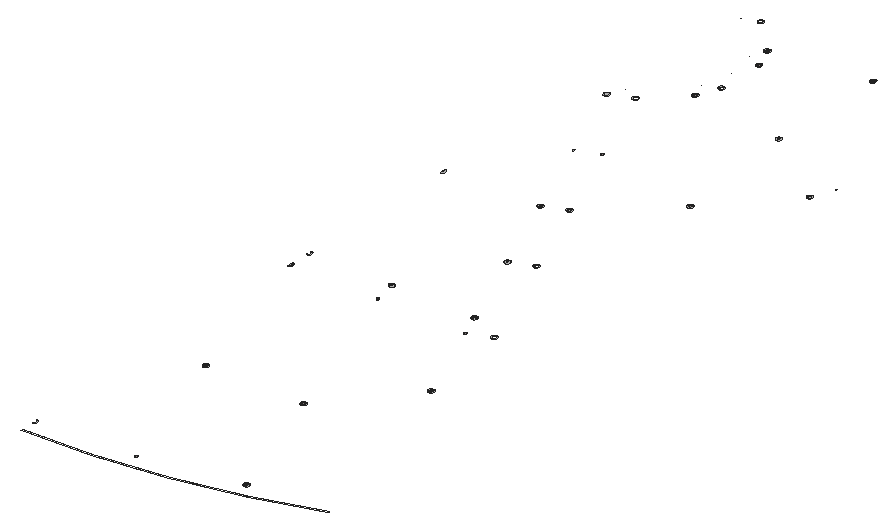
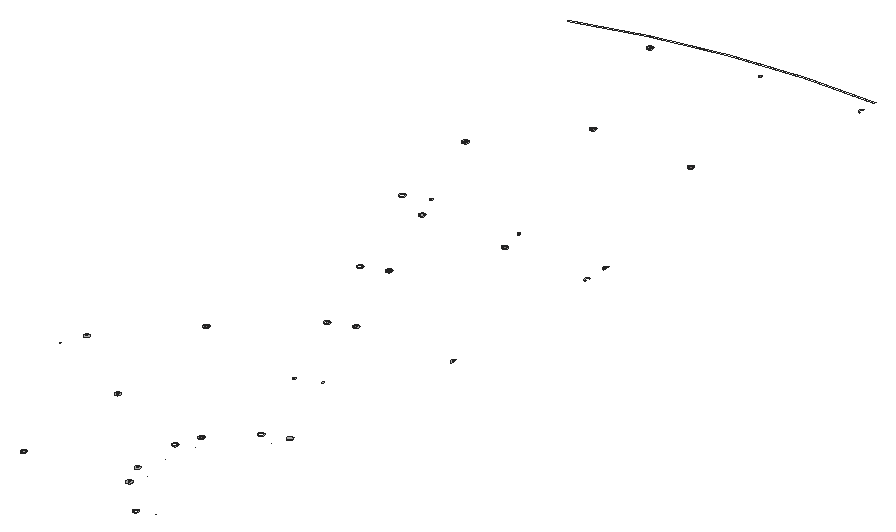
# SketchUp Ruby script. Lengths in inches.
U = 1.inch
M = Sketchup.active_model
def pt(a) = Geom::Point3d.new(a.map { |v| v * U })
def face(e, loops, mat)
  f = e.add_face(loops[0].map { |a| pt(a) })
  loops[1..].each { |l| e.add_face(l.map { |a| pt(a) }).erase! }
  f.material = f.back_material = mat if mat
  f
end
# faces: each face lists its corners as indices into pts; further lists are holes
def faces(e, pts, list, mat = nil) = list.each { |f| face(e, (f[0].is_a?(Array) ? f : [f]).map { |l| l.map { |i| pts[i] } }, mat) }
# xy, xz, yz: faces in a plane at the given z, y or x. An outline is a flat list of corners, or four numbers for a rectangle; further outlines are holes
def ring(l) = l.size == 4 ? [[l[0], l[1]], [l[2], l[1]], [l[2], l[3]], [l[0], l[3]]] : l.each_slice(2).to_a
def flat(e, list, mat, &to3) = list.each { |f| face(e, (f[0].is_a?(Array) ? f : [f]).map { |l| ring(l).map { |u, v| to3.(u, v) } }, mat) }
def xy(e, z, list, mat = nil) = flat(e, list, mat) { |x, y| [x, y, z] }
def xz(e, y, list, mat = nil) = flat(e, list, mat) { |x, z| [x, y, z] }
def yz(e, x, list, mat = nil) = flat(e, list, mat) { |y, z| [x, y, z] }
def lines(e, pts, list) = list.each { |a, b| e.add_line(pt(pts[a]), pt(pts[b])) }
# prism: a flat outline (further loops are holes) pulled along v
def prism(e, loops, v, mat = nil)
  f = face(e, loops, mat); d = Geom::Vector3d.new(v.map { |x| x * U })
  f.pushpull(f.normal.samedirection?(d) ? d.length : -d.length)
end
def box(e, o, s, mat = nil) = prism(e, [[o, [o[0] + s[0], o[1], o[2]], [o[0] + s[0], o[1] + s[1], o[2]], [o[0], o[1] + s[1], o[2]]]], [0, 0, s[2]], mat)
def at(x, y, z, deg = 0) = Geom::Transformation.translation(pt([x, y, z])) * Geom::Transformation.rotation(ORIGIN, Z_AXIS, deg.degrees)
def axes(o, x, y, z) = Geom::Transformation.new([*x, 0, *y, 0, *z, 0, *pt(o).to_a, 1])
def part(name) = M.definitions.add(name)
# library, detail: a bought-in or finely detailed component or shape, given as its bounding box
def library(name, o, s) = part(name).tap { |d| box(d.entities, o, s) }
def detail(e, o, s) = box(e.add_group.entities, o, s)
def put(e, d, t, mat = nil) = e.add_instance(d, t).tap { |i| i.material = mat if mat }
def group(e, t, mat = nil) = e.add_group.tap { |g| g.transformation = t; g.material = mat if mat }.entities
root = M.entities
M.materials.add("[Asphalt_Stamped_Brick]").color = [149, 133, 134]
M.materials.add("[Metal_Steel_Textured_White]").color = [191, 191, 191]
xy(root,3.625,[[153.108,137.349,153.103,137.35,153.098,137.352,153.094,137.355,153.09,137.359,153.088,137.364,153.088,137.374,153.09,137.379,153.098,137.387,153.103,137.389,153.113,137.389,153.118,137.387,153.122,137.383,153.125,137.379,153.127,137.374,153.128,137.369,153.127,137.364,153.125,137.359,153.122,137.355,153.118,137.352,153.113,137.35],[156.34,137.968,156.336,137.97,156.331,137.974,156.328,137.978,156.326,137.983,156.326,137.993,156.328,137.998,156.331,138.002,156.336,138.005,156.34,138.007,156.345,138.008,156.351,138.007,156.355,138.005,156.36,138.002,156.363,137.998,156.365,137.993,156.365,137.983,156.363,137.978,156.36,137.974,156.355,137.97,156.351,137.968],[151.473,142.332,151.468,142.333,151.463,142.335,151.459,142.338,151.456,142.342,151.454,142.347,151.453,142.352,151.454,142.357,151.456,142.362,151.459,142.366,151.463,142.369,151.468,142.371,151.473,142.372,151.478,142.371,151.483,142.369,151.487,142.366,151.491,142.362,151.493,142.357,151.493,142.347,151.491,142.342,151.487,142.338,151.483,142.335,151.478,142.333],[154.784,142.332,154.779,142.333,154.774,142.335,154.77,142.338,154.767,142.342,154.765,142.347,154.764,142.352,154.765,142.357,154.767,142.362,154.77,142.366,154.774,142.369,154.779,142.371,154.784,142.372,154.789,142.371,154.794,142.369,154.798,142.366,154.801,142.362,154.803,142.357,154.804,142.352,154.803,142.347,154.801,142.342,154.798,142.338,154.794,142.335,154.789,142.333],[156.99,144.988,156.985,144.99,156.981,144.993,156.978,144.998,156.976,145.002,156.975,145.008,156.976,145.013,156.978,145.018,156.981,145.022,156.985,145.025,156.99,145.027,156.995,145.028,157,145.027,157.005,145.025,157.009,145.022,157.012,145.018,157.014,145.013,157.015,145.008,157.014,145.002,157.012,144.998,157.009,144.993,157.005,144.99,157,144.988],
  [152.78,147.988,152.775,147.99,152.771,147.993,152.768,147.998,152.766,148.002,152.765,148.008,152.766,148.013,152.768,148.018,152.771,148.022,152.775,148.025,152.78,148.027,152.79,148.027,152.795,148.025,152.799,148.022,152.802,148.018,152.804,148.013,152.805,148.008,152.804,148.002,152.802,147.998,152.799,147.993,152.795,147.99,152.79,147.988],[155.747,147.988,155.742,147.99,155.738,147.993,155.735,147.998,155.733,148.002,155.732,148.008,155.733,148.013,155.735,148.018,155.738,148.022,155.742,148.025,155.747,148.027,155.757,148.027,155.762,148.025,155.766,148.022,155.769,148.018,155.771,148.013,155.772,148.008,155.771,148.002,155.769,147.998,155.766,147.993,155.762,147.99,155.757,147.988],[152.62,148.786,152.615,148.787,152.61,148.789,152.606,148.792,152.602,148.796,152.6,148.801,152.6,148.811,152.602,148.816,152.606,148.82,152.61,148.823,152.615,148.825,152.62,148.826,152.625,148.825,152.63,148.823,152.634,148.82,152.637,148.816,152.639,148.811,152.64,148.806,152.639,148.801,152.637,148.796,152.634,148.792,152.63,148.789,152.625,148.787],[153.011,154.594,153.006,154.596,153.002,154.599,152.999,154.604,152.997,154.608,152.996,154.614,152.997,154.619,152.999,154.624,153.002,154.628,153.006,154.631,153.011,154.633,153.021,154.633,153.026,154.631,153.03,154.628,153.033,154.624,153.035,154.619,153.036,154.614,153.035,154.608,153.033,154.604,153.03,154.599,153.026,154.596,153.021,154.594],[156.122,157.053,156.117,157.054,156.112,157.056,156.108,157.059,156.105,157.063,156.103,157.068,156.102,157.073,156.103,157.078,156.105,157.083,156.108,157.087,156.112,157.09,156.117,157.092,156.122,157.093,156.128,157.092,156.132,157.09,156.136,157.087,156.14,157.083,156.142,157.078,156.142,157.068,156.14,157.063,156.136,157.059,156.132,157.056,156.128,157.054],
  [152.551,157.803,152.546,157.804,152.541,157.806,152.537,157.809,152.533,157.813,152.531,157.818,152.531,157.828,152.533,157.833,152.537,157.837,152.541,157.84,152.546,157.842,152.551,157.843,152.556,157.842,152.561,157.84,152.565,157.837,152.568,157.833,152.57,157.828,152.571,157.823,152.57,157.818,152.568,157.813,152.565,157.809,152.561,157.806,152.556,157.804],[158.582,160.159,158.577,160.16,158.572,160.162,158.568,160.165,158.564,160.169,158.5625,160.174,158.562,160.179,158.5625,160.185,158.564,160.189,158.568,160.194,158.572,160.197,158.577,160.199,158.587,160.199,158.592,160.197,158.596,160.194,158.599,160.189,158.601,160.185,158.602,160.179,158.601,160.174,158.599,160.169,158.596,160.165,158.592,160.162,158.587,160.16],[155.678,161.362,155.673,161.363,155.668,161.365,155.664,161.368,155.661,161.372,155.659,161.377,155.658,161.382,155.659,161.387,155.661,161.392,155.664,161.396,155.668,161.399,155.673,161.401,155.678,161.402,155.683,161.401,155.688,161.399,155.692,161.396,155.695,161.392,155.697,161.387,155.698,161.382,155.697,161.377,155.695,161.372,155.692,161.368,155.688,161.365,155.683,161.363],[152.469,161.827,152.463,161.828,152.459,161.83,152.455,161.833,152.451,161.837,152.449,161.842,152.449,161.852,152.451,161.857,152.459,161.865,152.463,161.867,152.474,161.867,152.479,161.865,152.483,161.861,152.486,161.857,152.488,161.852,152.489,161.847,152.488,161.842,152.486,161.837,152.483,161.833,152.479,161.83,152.474,161.828],[152.774,164.15,152.769,164.151,152.764,164.153,152.76,164.156,152.757,164.16,152.755,164.165,152.754,164.17,152.755,164.175,152.757,164.18,152.76,164.184,152.764,164.187,152.769,164.189,152.774,164.19,152.779,164.189,152.784,164.187,152.788,164.184,152.791,164.18,152.793,164.175,152.794,164.17,152.793,164.165,152.791,164.16,152.788,164.156,152.784,164.153,152.779,164.151]],"[Asphalt_Stamped_Brick]")
xy(root,3.625,[[149.818,137.073,149.818,137.074,149.841,137.077,149.862,137.086,149.88,137.1,149.894,137.118,149.903,137.139,149.906,137.162,149.903,137.185,149.894,137.206,149.88,137.224,149.862,137.238,149.841,137.247,149.818,137.25,149.818,137.251,149.841,137.248,149.862,137.239,149.881,137.225,149.895,137.207,149.904,137.185,149.907,137.162,149.904,137.139,149.895,137.118,149.881,137.099,149.862,137.085,149.841,137.076],[[153.108,137.333,153.098,137.334,153.089,137.338,153.082,137.343,153.076,137.351,153.072,137.36,153.071,137.369,153.072,137.379,153.076,137.388,153.082,137.395,153.089,137.401,153.098,137.405,153.108,137.406,153.117,137.405,153.126,137.401,153.134,137.395,153.139,137.388,153.143,137.379,153.144,137.369,153.143,137.36,153.139,137.351,153.134,137.343,153.126,137.338,153.117,137.334],[153.108,137.349,153.113,137.35,153.118,137.352,153.122,137.355,153.125,137.359,153.127,137.364,153.128,137.369,153.127,137.374,153.125,137.379,153.122,137.383,153.118,137.387,153.113,137.389,153.103,137.389,153.098,137.387,153.09,137.379,153.088,137.374,153.088,137.364,153.09,137.359,153.094,137.355,153.098,137.352,153.103,137.35]],[[156.345,137.899,156.322,137.902,156.301,137.911,156.283,137.925,156.269,137.943,156.26,137.965,156.257,137.988,156.26,138.011,156.269,138.032,156.283,138.051,156.301,138.065,156.322,138.074,156.345,138.077,156.368,138.074,156.39,138.065,156.408,138.051,156.422,138.032,156.431,138.011,156.434,137.988,156.431,137.965,156.422,137.943,156.408,137.925,156.39,137.911,156.368,137.902],[156.345,137.9,156.368,137.903,156.389,137.912,156.408,137.926,156.422,137.944,156.43,137.965,156.433,137.988,156.43,138.011,156.422,138.032,156.408,138.05,156.389,138.064,156.368,138.073,156.345,138.076,156.323,138.073,156.302,138.064,156.283,138.05,156.269,138.032,156.261,138.011,156.258,137.988,156.261,137.965,156.269,137.944,156.283,137.926,156.302,137.912,156.323,137.903]],[[156.345,137.9,156.323,137.903,156.302,137.912,156.283,137.926,156.269,137.944,156.261,137.965,156.258,137.988,156.261,138.011,156.269,138.032,156.283,138.05,156.302,138.064,156.323,138.073,156.345,138.076,156.368,138.073,156.389,138.064,156.408,138.05,156.422,138.032,156.43,138.011,156.433,137.988,156.43,137.965,156.422,137.944,156.408,137.926,156.389,137.912,156.368,137.903],[156.345,137.951,156.355,137.952,156.364,137.956,156.371,137.962,156.377,137.969,156.381,137.978,156.382,137.988,156.381,137.997,156.377,138.006,156.371,138.014,156.364,138.019,156.355,138.023,156.345,138.024,156.336,138.023,156.327,138.019,156.32,138.014,156.314,138.006,156.31,137.997,156.309,137.988,156.31,137.978,156.314,137.969,156.32,137.962,156.327,137.956,156.336,137.952]],[[156.345,137.951,156.336,137.952,156.327,137.956,156.32,137.962,156.314,137.969,156.31,137.978,156.309,137.988,156.31,137.997,156.314,138.006,156.32,138.014,156.327,138.019,156.336,138.023,156.345,138.024,156.355,138.023,156.364,138.019,156.371,138.014,156.377,138.006,156.381,137.997,156.382,137.988,156.381,137.978,156.377,137.969,156.371,137.962,156.364,137.956,156.355,137.952],[156.34,137.968,156.351,137.968,156.355,137.97,156.36,137.974,156.363,137.978,156.365,137.983,156.365,137.993,156.363,137.998,156.36,138.002,156.355,138.005,156.351,138.007,156.345,138.008,156.34,138.007,156.336,138.005,156.331,138.002,156.328,137.998,156.326,137.993,156.326,137.983,156.328,137.978,156.331,137.974,156.336,137.97]],
  [[151.473,142.263,151.45,142.266,151.429,142.275,151.41,142.289,151.396,142.307,151.387,142.329,151.384,142.352,151.387,142.375,151.396,142.396,151.41,142.415,151.429,142.429,151.45,142.438,151.473,142.441,151.496,142.438,151.518,142.429,151.536,142.415,151.55,142.396,151.559,142.375,151.562,142.352,151.559,142.329,151.55,142.307,151.536,142.289,151.518,142.275,151.496,142.266],[151.473,142.264,151.496,142.267,151.517,142.276,151.535,142.29,151.549,142.308,151.558,142.329,151.561,142.352,151.558,142.375,151.549,142.396,151.535,142.414,151.517,142.428,151.496,142.437,151.473,142.44,151.451,142.437,151.429,142.428,151.411,142.414,151.397,142.396,151.388,142.375,151.385,142.352,151.388,142.329,151.397,142.308,151.411,142.29,151.429,142.276,151.451,142.267]],[[154.784,142.263,154.761,142.266,154.74,142.275,154.721,142.289,154.707,142.307,154.698,142.329,154.695,142.352,154.698,142.375,154.707,142.396,154.721,142.415,154.74,142.429,154.761,142.438,154.784,142.441,154.807,142.438,154.828,142.429,154.847,142.415,154.861,142.396,154.87,142.375,154.873,142.352,154.87,142.329,154.861,142.307,154.847,142.289,154.828,142.275,154.807,142.266],[154.784,142.264,154.807,142.267,154.828,142.276,154.846,142.29,154.86,142.308,154.869,142.329,154.872,142.352,154.869,142.375,154.86,142.396,154.846,142.414,154.828,142.428,154.807,142.437,154.784,142.44,154.761,142.437,154.74,142.428,154.722,142.414,154.708,142.396,154.699,142.375,154.696,142.352,154.699,142.329,154.708,142.308,154.722,142.29,154.74,142.276,154.761,142.267]],[[151.473,142.264,151.451,142.267,151.429,142.276,151.411,142.29,151.397,142.308,151.388,142.329,151.385,142.352,151.388,142.375,151.397,142.396,151.411,142.414,151.429,142.428,151.451,142.437,151.473,142.44,151.496,142.437,151.517,142.428,151.535,142.414,151.549,142.396,151.558,142.375,151.561,142.352,151.558,142.329,151.549,142.308,151.535,142.29,151.517,142.276,151.496,142.267],[151.473,142.315,151.483,142.317,151.492,142.32,151.499,142.326,151.505,142.334,151.509,142.342,151.51,142.352,151.509,142.361,151.505,142.37,151.499,142.378,151.492,142.384,151.483,142.387,151.473,142.389,151.464,142.387,151.455,142.384,151.447,142.378,151.442,142.37,151.438,142.361,151.437,142.352,151.438,142.342,151.442,142.334,151.447,142.326,151.455,142.32,151.464,142.317]],[[151.473,142.315,151.464,142.317,151.455,142.32,151.447,142.326,151.442,142.334,151.438,142.342,151.437,142.352,151.438,142.361,151.442,142.37,151.447,142.378,151.455,142.384,151.464,142.387,151.473,142.389,151.483,142.387,151.492,142.384,151.499,142.378,151.505,142.37,151.509,142.361,151.51,142.352,151.509,142.342,151.505,142.334,151.499,142.326,151.492,142.32,151.483,142.317],[151.473,142.332,151.478,142.333,151.483,142.335,151.487,142.338,151.491,142.342,151.493,142.347,151.493,142.357,151.491,142.362,151.487,142.366,151.483,142.369,151.478,142.371,151.473,142.372,151.468,142.371,151.463,142.369,151.459,142.366,151.456,142.362,151.454,142.357,151.453,142.352,151.454,142.347,151.456,142.342,151.459,142.338,151.463,142.335,151.468,142.333]],[[154.784,142.315,154.775,142.317,154.766,142.32,154.758,142.326,154.752,142.334,154.749,142.342,154.747,142.352,154.749,142.361,154.752,142.37,154.758,142.378,154.766,142.384,154.775,142.387,154.784,142.389,154.794,142.387,154.802,142.384,154.81,142.378,154.816,142.37,154.819,142.361,154.821,142.352,154.819,142.342,154.816,142.334,154.81,142.326,154.802,142.32,154.794,142.317],[154.784,142.332,154.789,142.333,154.794,142.335,154.798,142.338,154.801,142.342,154.803,142.347,154.804,142.352,154.803,142.357,154.801,142.362,154.798,142.366,154.794,142.369,154.789,142.371,154.784,142.372,154.779,142.371,154.774,142.369,154.77,142.366,154.767,142.362,154.765,142.357,154.764,142.352,154.765,142.347,154.767,142.342,154.77,142.338,154.774,142.335,154.779,142.333]],
  [[156.995,144.919,156.972,144.922,156.95,144.931,156.932,144.945,156.918,144.963,156.909,144.985,156.906,145.008,156.909,145.031,156.918,145.052,156.932,145.07,156.95,145.085,156.972,145.093,156.995,145.096,157.018,145.093,157.039,145.085,157.058,145.07,157.072,145.052,157.081,145.031,157.084,145.008,157.081,144.985,157.072,144.963,157.058,144.945,157.039,144.931,157.018,144.922],[156.995,144.92,157.018,144.923,157.039,144.931,157.057,144.945,157.071,144.964,157.08,144.985,157.083,145.008,157.08,145.03,157.071,145.052,157.057,145.07,157.039,145.084,157.018,145.092,156.995,145.095,156.972,145.092,156.951,145.084,156.933,145.07,156.919,145.052,156.91,145.03,156.907,145.008,156.91,144.985,156.919,144.964,156.933,144.945,156.951,144.931,156.972,144.923]],[[156.995,144.971,156.985,144.972,156.977,144.976,156.969,144.982,156.963,144.989,156.959,144.998,156.958,145.008,156.959,145.017,156.963,145.026,156.969,145.033,156.977,145.039,156.985,145.043,156.995,145.044,157.004,145.043,157.013,145.039,157.021,145.033,157.027,145.026,157.03,145.017,157.031,145.008,157.03,144.998,157.027,144.989,157.021,144.982,157.013,144.976,157.004,144.972],[156.99,144.988,157,144.988,157.005,144.99,157.009,144.993,157.012,144.998,157.014,145.002,157.015,145.008,157.014,145.013,157.012,145.018,157.009,145.022,157.005,145.025,157,145.027,156.995,145.028,156.99,145.027,156.985,145.025,156.981,145.022,156.978,145.018,156.976,145.013,156.975,145.008,156.976,145.002,156.978,144.998,156.981,144.993,156.985,144.99]],[149.818,147.919,149.818,147.92,149.841,147.923,149.862,147.931,149.88,147.945,149.894,147.964,149.903,147.985,149.906,148.008,149.903,148.03,149.894,148.051,149.88,148.07,149.862,148.084,149.841,148.092,149.818,148.095,149.818,148.096,149.841,148.093,149.862,148.085,149.881,148.07,149.895,148.052,149.904,148.031,149.907,148.008,149.904,147.985,149.895,147.963,149.881,147.945,149.862,147.931,149.841,147.922],[[152.785,147.971,152.776,147.972,152.767,147.976,152.759,147.982,152.753,147.989,152.75,147.998,152.748,148.008,152.75,148.017,152.753,148.026,152.759,148.033,152.767,148.039,152.776,148.043,152.785,148.044,152.795,148.043,152.803,148.039,152.811,148.033,152.817,148.026,152.82,148.017,152.822,148.008,152.82,147.998,152.817,147.989,152.811,147.982,152.803,147.976,152.795,147.972],[152.78,147.988,152.79,147.988,152.795,147.99,152.799,147.993,152.802,147.998,152.804,148.002,152.805,148.008,152.804,148.013,152.802,148.018,152.799,148.022,152.795,148.025,152.79,148.027,152.78,148.027,152.775,148.025,152.771,148.022,152.768,148.018,152.766,148.013,152.765,148.008,152.766,148.002,152.768,147.998,152.771,147.993,152.775,147.99]],[[155.752,147.971,155.743,147.972,155.734,147.976,155.726,147.982,155.721,147.989,155.717,147.998,155.716,148.008,155.717,148.017,155.721,148.026,155.726,148.033,155.734,148.039,155.743,148.043,155.752,148.044,155.762,148.043,155.771,148.039,155.778,148.033,155.784,148.026,155.788,148.017,155.789,148.008,155.788,147.998,155.784,147.989,155.778,147.982,155.771,147.976,155.762,147.972],[155.747,147.988,155.757,147.988,155.762,147.99,155.766,147.993,155.769,147.998,155.771,148.002,155.772,148.008,155.771,148.013,155.769,148.018,155.766,148.022,155.762,148.025,155.757,148.027,155.747,148.027,155.742,148.025,155.738,148.022,155.735,148.018,155.733,148.013,155.732,148.008,155.733,148.002,155.735,147.998,155.738,147.993,155.742,147.99]],
  [149.818,147.988,149.818,148.027,149.823,148.027,149.828,148.025,149.832,148.022,149.835,148.018,149.837,148.013,149.838,148.008,149.837,148.002,149.835,147.998,149.832,147.993,149.828,147.99,149.823,147.988],[[156.49,148.224,156.467,148.227,156.445,148.236,156.427,148.25,156.413,148.269,156.404,148.29,156.401,148.313,156.404,148.336,156.413,148.358,156.427,148.376,156.445,148.39,156.467,148.399,156.49,148.402,156.513,148.399,156.534,148.39,156.553,148.376,156.567,148.358,156.576,148.336,156.579,148.313,156.576,148.29,156.567,148.269,156.553,148.25,156.534,148.236,156.513,148.227],[156.49,148.225,156.513,148.228,156.534,148.237,156.552,148.251,156.566,148.269,156.575,148.29,156.578,148.313,156.575,148.336,156.566,148.357,156.552,148.375,156.534,148.389,156.513,148.398,156.49,148.401,156.467,148.398,156.446,148.389,156.428,148.375,156.414,148.357,156.405,148.336,156.402,148.313,156.405,148.29,156.414,148.269,156.428,148.251,156.446,148.237,156.467,148.228]],[149.818,148.717,149.818,148.718,149.841,148.721,149.862,148.73,149.88,148.744,149.894,148.762,149.903,148.783,149.906,148.806,149.903,148.829,149.894,148.85,149.88,148.868,149.862,148.882,149.841,148.891,149.818,148.894,149.818,148.895,149.841,148.892,149.862,148.883,149.881,148.869,149.895,148.85,149.904,148.829,149.907,148.806,149.904,148.783,149.895,148.762,149.881,148.743,149.862,148.729,149.841,148.72],[[152.62,148.717,152.597,148.72,152.575,148.729,152.557,148.743,152.543,148.762,152.534,148.783,152.531,148.806,152.534,148.829,152.543,148.85,152.557,148.869,152.575,148.883,152.597,148.892,152.62,148.895,152.643,148.892,152.664,148.883,152.683,148.869,152.697,148.85,152.706,148.829,152.709,148.806,152.706,148.783,152.697,148.762,152.683,148.743,152.664,148.729,152.643,148.72],[152.62,148.718,152.642,148.721,152.664,148.73,152.682,148.744,152.696,148.762,152.705,148.783,152.708,148.806,152.705,148.829,152.696,148.85,152.682,148.868,152.664,148.882,152.642,148.891,152.62,148.894,152.597,148.891,152.576,148.882,152.558,148.868,152.544,148.85,152.535,148.829,152.532,148.806,152.535,148.783,152.544,148.762,152.558,148.744,152.576,148.73,152.597,148.721]],[[155.421,148.717,155.398,148.72,155.377,148.729,155.359,148.743,155.345,148.762,155.336,148.783,155.333,148.806,155.336,148.829,155.345,148.85,155.359,148.869,155.377,148.883,155.398,148.892,155.421,148.895,155.444,148.892,155.466,148.883,155.484,148.869,155.498,148.85,155.507,148.829,155.51,148.806,155.507,148.783,155.498,148.762,155.484,148.743,155.466,148.729,155.444,148.72],[155.421,148.718,155.444,148.721,155.465,148.73,155.484,148.744,155.498,148.762,155.506,148.783,155.509,148.806,155.506,148.829,155.498,148.85,155.484,148.868,155.465,148.882,155.444,148.891,155.421,148.894,155.399,148.891,155.378,148.882,155.359,148.868,155.345,148.85,155.337,148.829,155.334,148.806,155.337,148.783,155.345,148.762,155.359,148.744,155.378,148.73,155.399,148.721]],
  [[152.62,148.718,152.597,148.721,152.576,148.73,152.558,148.744,152.544,148.762,152.535,148.783,152.532,148.806,152.535,148.829,152.544,148.85,152.558,148.868,152.576,148.882,152.597,148.891,152.62,148.894,152.642,148.891,152.664,148.882,152.682,148.868,152.696,148.85,152.705,148.829,152.708,148.806,152.705,148.783,152.696,148.762,152.682,148.744,152.664,148.73,152.642,148.721],[152.62,148.769,152.629,148.771,152.638,148.774,152.646,148.78,152.651,148.788,152.655,148.796,152.656,148.806,152.655,148.815,152.651,148.824,152.646,148.832,152.638,148.838,152.629,148.841,152.62,148.843,152.61,148.841,152.601,148.838,152.594,148.832,152.588,148.824,152.584,148.815,152.583,148.806,152.584,148.796,152.588,148.788,152.594,148.78,152.601,148.774,152.61,148.771]],[[155.421,148.718,155.399,148.721,155.378,148.73,155.359,148.744,155.345,148.762,155.337,148.783,155.334,148.806,155.337,148.829,155.345,148.85,155.359,148.868,155.378,148.882,155.399,148.891,155.421,148.894,155.444,148.891,155.465,148.882,155.484,148.868,155.498,148.85,155.506,148.829,155.509,148.806,155.506,148.783,155.498,148.762,155.484,148.744,155.465,148.73,155.444,148.721],[155.421,148.769,155.431,148.771,155.44,148.774,155.447,148.78,155.453,148.788,155.457,148.796,155.458,148.806,155.457,148.815,155.453,148.824,155.447,148.832,155.44,148.838,155.431,148.841,155.421,148.843,155.412,148.841,155.403,148.838,155.396,148.832,155.39,148.824,155.386,148.815,155.385,148.806,155.386,148.796,155.39,148.788,155.396,148.78,155.403,148.774,155.412,148.771]],[[152.62,148.769,152.61,148.771,152.601,148.774,152.594,148.78,152.588,148.788,152.584,148.796,152.583,148.806,152.584,148.815,152.588,148.824,152.594,148.832,152.601,148.838,152.61,148.841,152.62,148.843,152.629,148.841,152.638,148.838,152.646,148.832,152.651,148.824,152.655,148.815,152.656,148.806,152.655,148.796,152.651,148.788,152.646,148.78,152.638,148.774,152.629,148.771],[152.62,148.786,152.625,148.787,152.63,148.789,152.634,148.792,152.637,148.796,152.639,148.801,152.64,148.806,152.639,148.811,152.637,148.816,152.634,148.82,152.63,148.823,152.625,148.825,152.62,148.826,152.615,148.825,152.61,148.823,152.606,148.82,152.602,148.816,152.6,148.811,152.6,148.801,152.602,148.796,152.606,148.792,152.61,148.789,152.615,148.787]],[[155.421,148.769,155.412,148.771,155.403,148.774,155.396,148.78,155.39,148.788,155.386,148.796,155.385,148.806,155.386,148.815,155.39,148.824,155.396,148.832,155.403,148.838,155.412,148.841,155.421,148.843,155.431,148.841,155.44,148.838,155.447,148.832,155.453,148.824,155.457,148.815,155.458,148.806,155.457,148.796,155.453,148.788,155.447,148.78,155.44,148.774,155.431,148.771],[155.421,148.786,155.427,148.787,155.431,148.789,155.436,148.792,155.439,148.796,155.441,148.801,155.441,148.811,155.439,148.816,155.436,148.82,155.431,148.823,155.427,148.825,155.421,148.826,155.416,148.825,155.412,148.823,155.407,148.82,155.404,148.816,155.402,148.811,155.402,148.801,155.404,148.796,155.407,148.792,155.412,148.789,155.416,148.787]],[[154.219,151.621,154.196,151.624,154.174,151.633,154.156,151.647,154.142,151.665,154.133,151.687,154.13,151.71,154.133,151.733,154.142,151.754,154.156,151.773,154.174,151.787,154.196,151.796,154.219,151.799,154.242,151.796,154.263,151.787,154.282,151.773,154.296,151.754,154.305,151.733,154.308,151.71,154.305,151.687,154.296,151.665,154.282,151.647,154.263,151.633,154.242,151.624],[154.219,151.622,154.241,151.625,154.263,151.634,154.281,151.648,154.295,151.666,154.304,151.687,154.307,151.71,154.304,151.733,154.295,151.754,154.281,151.772,154.263,151.786,154.241,151.795,154.219,151.798,154.196,151.795,154.175,151.786,154.157,151.772,154.143,151.754,154.134,151.733,154.131,151.71,154.134,151.687,154.143,151.666,154.157,151.648,154.175,151.634,154.196,151.625]],
  [[154.219,151.622,154.196,151.625,154.175,151.634,154.157,151.648,154.143,151.666,154.134,151.687,154.131,151.71,154.134,151.733,154.143,151.754,154.157,151.772,154.175,151.786,154.196,151.795,154.219,151.798,154.241,151.795,154.263,151.786,154.281,151.772,154.295,151.754,154.304,151.733,154.307,151.71,154.304,151.687,154.295,151.666,154.281,151.648,154.263,151.634,154.241,151.625],[154.219,151.673,154.228,151.674,154.237,151.678,154.245,151.684,154.25,151.691,154.254,151.7,154.255,151.71,154.254,151.719,154.25,151.728,154.245,151.736,154.237,151.741,154.228,151.745,154.219,151.746,154.209,151.745,154.2,151.741,154.193,151.736,154.187,151.728,154.183,151.719,154.182,151.71,154.183,151.7,154.187,151.691,154.193,151.684,154.2,151.678,154.209,151.674]],[[154.219,151.673,154.209,151.674,154.2,151.678,154.193,151.684,154.187,151.691,154.183,151.7,154.182,151.71,154.183,151.719,154.187,151.728,154.193,151.736,154.2,151.741,154.209,151.745,154.219,151.746,154.228,151.745,154.237,151.741,154.245,151.736,154.25,151.728,154.254,151.719,154.255,151.71,154.254,151.7,154.25,151.691,154.245,151.684,154.237,151.678,154.228,151.674],[154.214,151.69,154.224,151.69,154.229,151.692,154.233,151.696,154.236,151.7,154.238,151.705,154.239,151.71,154.238,151.715,154.236,151.72,154.233,151.724,154.229,151.727,154.224,151.729,154.219,151.73,154.214,151.729,154.209,151.727,154.205,151.724,154.201,151.72,154.199,151.715,154.199,151.705,154.201,151.7,154.209,151.692]],[154.214,151.69,154.209,151.692,154.201,151.7,154.199,151.705,154.199,151.715,154.201,151.72,154.205,151.724,154.209,151.727,154.214,151.729,154.219,151.73,154.224,151.729,154.229,151.727,154.233,151.724,154.236,151.72,154.238,151.715,154.239,151.71,154.238,151.705,154.236,151.7,154.233,151.696,154.229,151.692,154.224,151.69],[[154.956,151.926,154.933,151.929,154.912,151.938,154.893,151.952,154.879,151.971,154.87,151.992,154.867,152.015,154.87,152.038,154.879,152.06,154.893,152.078,154.912,152.092,154.933,152.101,154.956,152.104,154.979,152.101,155.001,152.092,155.019,152.078,155.033,152.06,155.042,152.038,155.045,152.015,155.042,151.992,155.033,151.971,155.019,151.952,155.001,151.938,154.979,151.929],[154.956,151.927,154.979,151.93,155,151.939,155.019,151.953,155.032,151.971,155.041,151.993,155.044,152.015,155.041,152.038,155.032,152.059,155.019,152.077,155,152.091,154.979,152.1,154.956,152.103,154.934,152.1,154.912,152.091,154.894,152.077,154.88,152.059,154.871,152.038,154.868,152.015,154.871,151.993,154.88,151.971,154.894,151.953,154.912,151.939,154.934,151.93]],[149.818,154.374,149.818,154.425,149.827,154.426,149.836,154.43,149.844,154.436,149.85,154.443,149.853,154.452,149.854,154.462,149.853,154.471,149.85,154.48,149.844,154.487,149.836,154.493,149.827,154.497,149.818,154.498,149.818,154.549,149.841,154.546,149.862,154.538,149.88,154.524,149.894,154.506,149.903,154.484,149.906,154.462,149.903,154.439,149.894,154.418,149.88,154.399,149.862,154.385,149.841,154.377],
  [149.818,154.442,149.818,154.482,149.823,154.481,149.828,154.479,149.832,154.476,149.835,154.472,149.837,154.467,149.838,154.462,149.837,154.456,149.835,154.452,149.832,154.447,149.828,154.444,149.823,154.442],[[153.016,154.525,152.993,154.528,152.971,154.537,152.953,154.551,152.939,154.569,152.93,154.591,152.927,154.614,152.93,154.637,152.939,154.658,152.953,154.676,152.971,154.691,152.993,154.699,153.016,154.702,153.039,154.699,153.06,154.691,153.079,154.676,153.093,154.658,153.102,154.637,153.105,154.614,153.102,154.591,153.093,154.569,153.079,154.551,153.06,154.537,153.039,154.528],[153.016,154.526,153.039,154.529,153.06,154.537,153.078,154.551,153.092,154.57,153.101,154.591,153.104,154.614,153.101,154.636,153.092,154.657,153.078,154.676,153.06,154.69,153.039,154.698,153.016,154.701,152.993,154.698,152.972,154.69,152.954,154.676,152.94,154.657,152.931,154.636,152.928,154.614,152.931,154.591,152.94,154.57,152.954,154.551,152.972,154.537,152.993,154.529]],[[153.016,154.526,152.993,154.529,152.972,154.537,152.954,154.551,152.94,154.57,152.931,154.591,152.928,154.614,152.931,154.636,152.94,154.657,152.954,154.676,152.972,154.69,152.993,154.698,153.016,154.701,153.039,154.698,153.06,154.69,153.078,154.676,153.092,154.657,153.101,154.636,153.104,154.614,153.101,154.591,153.092,154.57,153.078,154.551,153.06,154.537,153.039,154.529],[153.016,154.577,153.025,154.578,153.034,154.582,153.042,154.588,153.048,154.595,153.051,154.604,153.052,154.614,153.051,154.623,153.048,154.632,153.042,154.639,153.034,154.645,153.025,154.649,153.016,154.65,153.006,154.649,152.998,154.645,152.99,154.639,152.984,154.632,152.981,154.623,152.979,154.614,152.981,154.604,152.984,154.595,152.99,154.588,152.998,154.582,153.006,154.578]],[[153.016,154.577,153.006,154.578,152.998,154.582,152.99,154.588,152.984,154.595,152.981,154.604,152.979,154.614,152.981,154.623,152.984,154.632,152.99,154.639,152.998,154.645,153.006,154.649,153.016,154.65,153.025,154.649,153.034,154.645,153.042,154.639,153.048,154.632,153.051,154.623,153.052,154.614,153.051,154.604,153.048,154.595,153.042,154.588,153.034,154.582,153.025,154.578],[153.011,154.594,153.021,154.594,153.026,154.596,153.03,154.599,153.033,154.604,153.035,154.608,153.036,154.614,153.035,154.619,153.033,154.624,153.03,154.628,153.026,154.631,153.021,154.633,153.011,154.633,153.006,154.631,153.002,154.628,152.999,154.624,152.997,154.619,152.996,154.614,152.997,154.608,152.999,154.604,153.002,154.599,153.006,154.596]],[[153.754,154.83,153.731,154.833,153.709,154.842,153.691,154.856,153.677,154.875,153.668,154.896,153.665,154.919,153.668,154.942,153.677,154.964,153.691,154.982,153.709,154.996,153.731,155.005,153.754,155.008,153.777,155.005,153.798,154.996,153.816,154.982,153.831,154.964,153.839,154.942,153.842,154.919,153.839,154.896,153.831,154.875,153.816,154.856,153.798,154.842,153.777,154.833],[153.754,154.831,153.776,154.834,153.798,154.843,153.816,154.857,153.83,154.875,153.838,154.896,153.841,154.919,153.838,154.942,153.83,154.963,153.816,154.981,153.798,154.995,153.776,155.004,153.754,155.007,153.731,155.004,153.71,154.995,153.691,154.981,153.677,154.963,153.669,154.942,153.666,154.919,153.669,154.896,153.677,154.875,153.691,154.857,153.71,154.843,153.731,154.834]],
  [153.754,154.899,153.748,154.9,153.744,154.902,153.739,154.905,153.736,154.909,153.734,154.914,153.734,154.924,153.736,154.929,153.739,154.933,153.744,154.936,153.748,154.938,153.754,154.939,153.759,154.938,153.764,154.936,153.768,154.933,153.771,154.929,153.773,154.924,153.774,154.919,153.773,154.914,153.771,154.909,153.768,154.905,153.764,154.902,153.759,154.9],[[156.122,156.984,156.099,156.987,156.078,156.996,156.06,157.01,156.045,157.029,156.037,157.05,156.033,157.073,156.037,157.096,156.045,157.117,156.06,157.136,156.078,157.15,156.099,157.159,156.122,157.162,156.145,157.159,156.167,157.15,156.185,157.136,156.199,157.117,156.208,157.096,156.211,157.073,156.208,157.05,156.199,157.029,156.185,157.01,156.167,156.996,156.145,156.987],[156.122,156.985,156.145,156.988,156.166,156.997,156.185,157.011,156.199,157.029,156.207,157.05,156.21,157.073,156.207,157.096,156.199,157.117,156.185,157.135,156.166,157.149,156.145,157.158,156.122,157.161,156.1,157.158,156.078,157.149,156.06,157.135,156.046,157.117,156.037,157.096,156.034,157.073,156.037,157.05,156.046,157.029,156.06,157.011,156.078,156.997,156.1,156.988]],[[156.122,156.985,156.1,156.988,156.078,156.997,156.06,157.011,156.046,157.029,156.037,157.05,156.034,157.073,156.037,157.096,156.046,157.117,156.06,157.135,156.078,157.149,156.1,157.158,156.122,157.161,156.145,157.158,156.166,157.149,156.185,157.135,156.199,157.117,156.207,157.096,156.21,157.073,156.207,157.05,156.199,157.029,156.185,157.011,156.166,156.997,156.145,156.988],[156.122,157.036,156.132,157.038,156.141,157.041,156.148,157.047,156.154,157.055,156.158,157.063,156.159,157.073,156.158,157.082,156.154,157.091,156.148,157.099,156.141,157.105,156.132,157.108,156.122,157.11,156.113,157.108,156.104,157.105,156.096,157.099,156.091,157.091,156.087,157.082,156.086,157.073,156.087,157.063,156.091,157.055,156.096,157.047,156.104,157.041,156.113,157.038]],[[156.122,157.036,156.113,157.038,156.104,157.041,156.096,157.047,156.091,157.055,156.087,157.063,156.086,157.073,156.087,157.082,156.091,157.091,156.096,157.099,156.104,157.105,156.113,157.108,156.122,157.11,156.132,157.108,156.141,157.105,156.148,157.099,156.154,157.091,156.158,157.082,156.159,157.073,156.158,157.063,156.154,157.055,156.148,157.047,156.141,157.041,156.132,157.038],[156.122,157.053,156.128,157.054,156.132,157.056,156.136,157.059,156.14,157.063,156.142,157.068,156.142,157.078,156.14,157.083,156.136,157.087,156.132,157.09,156.128,157.092,156.122,157.093,156.117,157.092,156.112,157.09,156.108,157.087,156.105,157.083,156.103,157.078,156.102,157.073,156.103,157.068,156.105,157.063,156.108,157.059,156.112,157.056,156.117,157.054]],[151.813,157.497,151.808,157.498,151.803,157.5,151.799,157.503,151.796,157.507,151.794,157.512,151.793,157.517,151.794,157.522,151.796,157.527,151.799,157.531,151.803,157.535,151.808,157.537,151.818,157.537,151.823,157.535,151.827,157.531,151.83,157.527,151.832,157.522,151.833,157.517,151.832,157.512,151.83,157.507,151.827,157.503,151.823,157.5,151.818,157.498],
  [[152.551,157.786,152.541,157.788,152.532,157.791,152.525,157.797,152.519,157.805,152.515,157.813,152.514,157.823,152.515,157.832,152.519,157.841,152.525,157.849,152.532,157.855,152.541,157.858,152.551,157.859,152.56,157.858,152.569,157.855,152.577,157.849,152.582,157.841,152.586,157.832,152.587,157.823,152.586,157.813,152.582,157.805,152.577,157.797,152.569,157.791,152.56,157.788],[152.551,157.803,152.556,157.804,152.561,157.806,152.565,157.809,152.568,157.813,152.57,157.818,152.571,157.823,152.57,157.828,152.568,157.833,152.565,157.837,152.561,157.84,152.556,157.842,152.551,157.843,152.546,157.842,152.541,157.84,152.537,157.837,152.533,157.833,152.531,157.828,152.531,157.818,152.533,157.813,152.537,157.809,152.541,157.806,152.546,157.804]],[[158.276,159.354,158.253,159.357,158.232,159.366,158.214,159.38,158.2,159.398,158.191,159.419,158.188,159.442,158.191,159.465,158.2,159.486,158.214,159.504,158.232,159.518,158.253,159.527,158.276,159.53,158.299,159.527,158.32,159.518,158.338,159.504,158.352,159.486,158.361,159.465,158.364,159.442,158.361,159.419,158.352,159.398,158.338,159.38,158.32,159.366,158.299,159.357],[158.276,159.405,158.286,159.406,158.295,159.41,158.302,159.416,158.308,159.423,158.312,159.432,158.313,159.442,158.312,159.451,158.308,159.46,158.302,159.468,158.295,159.473,158.286,159.477,158.276,159.478,158.267,159.477,158.258,159.473,158.25,159.468,158.245,159.46,158.241,159.451,158.24,159.442,158.241,159.432,158.245,159.423,158.25,159.416,158.258,159.41,158.267,159.406]],[[158.276,159.405,158.267,159.406,158.258,159.41,158.25,159.416,158.245,159.423,158.241,159.432,158.24,159.442,158.241,159.451,158.245,159.46,158.25,159.468,158.258,159.473,158.267,159.477,158.276,159.478,158.286,159.477,158.295,159.473,158.302,159.468,158.308,159.46,158.312,159.451,158.313,159.442,158.312,159.432,158.308,159.423,158.302,159.416,158.295,159.41,158.286,159.406],[158.271,159.422,158.281,159.422,158.286,159.424,158.294,159.432,158.296,159.437,158.296,159.447,158.294,159.452,158.29,159.456,158.286,159.459,158.281,159.461,158.276,159.462,158.271,159.461,158.266,159.459,158.262,159.456,158.259,159.452,158.257,159.447,158.256,159.442,158.257,159.437,158.259,159.432,158.262,159.428,158.266,159.424]],[[150.61,160.332,150.587,160.335,150.566,160.344,150.547,160.358,150.533,160.377,150.524,160.398,150.521,160.421,150.524,160.444,150.533,160.466,150.547,160.484,150.566,160.498,150.587,160.507,150.61,160.51,150.633,160.507,150.655,160.498,150.673,160.484,150.6875,160.466,150.696,160.444,150.699,160.421,150.696,160.398,150.6875,160.377,150.673,160.358,150.655,160.344,150.633,160.335],[150.61,160.333,150.633,160.336,150.654,160.345,150.672,160.359,150.686,160.377,150.695,160.398,150.698,160.421,150.695,160.444,150.686,160.465,150.672,160.483,150.654,160.497,150.633,160.506,150.61,160.509,150.588,160.506,150.566,160.497,150.548,160.483,150.534,160.465,150.525,160.444,150.522,160.421,150.525,160.398,150.534,160.377,150.548,160.359,150.566,160.345,150.588,160.336]],[[150.61,160.333,150.588,160.336,150.566,160.345,150.548,160.359,150.534,160.377,150.525,160.398,150.522,160.421,150.525,160.444,150.534,160.465,150.548,160.483,150.566,160.497,150.588,160.506,150.61,160.509,150.633,160.506,150.654,160.497,150.672,160.483,150.686,160.465,150.695,160.444,150.698,160.421,150.695,160.398,150.686,160.377,150.672,160.359,150.654,160.345,150.633,160.336],[150.61,160.385,150.62,160.386,150.629,160.389,150.636,160.395,150.642,160.403,150.646,160.412,150.647,160.421,150.646,160.431,150.642,160.439,150.636,160.447,150.629,160.453,150.62,160.456,150.61,160.458,150.601,160.456,150.592,160.453,150.584,160.447,150.579,160.439,150.575,160.431,150.574,160.421,150.575,160.412,150.579,160.403,150.584,160.395,150.592,160.389,150.601,160.386]],
  [[151.348,160.638,151.325,160.641,151.304,160.65,151.285,160.664,151.271,160.682,151.262,160.704,151.259,160.727,151.262,160.75,151.271,160.771,151.285,160.79,151.304,160.804,151.325,160.8125,151.348,160.816,151.371,160.8125,151.392,160.804,151.411,160.79,151.425,160.771,151.434,160.75,151.437,160.727,151.434,160.704,151.425,160.682,151.411,160.664,151.392,160.65,151.371,160.641],[151.348,160.639,151.371,160.642,151.392,160.651,151.41,160.664,151.424,160.683,151.433,160.704,151.436,160.727,151.433,160.749,151.424,160.771,151.41,160.789,151.392,160.803,151.371,160.812,151.348,160.815,151.325,160.812,151.304,160.803,151.286,160.789,151.272,160.771,151.263,160.749,151.26,160.727,151.263,160.704,151.272,160.683,151.286,160.664,151.304,160.651,151.325,160.642]],[[155.678,161.294,155.655,161.297,155.634,161.306,155.616,161.32,155.602,161.338,155.593,161.359,155.59,161.382,155.593,161.405,155.602,161.426,155.616,161.444,155.634,161.458,155.655,161.467,155.678,161.47,155.701,161.467,155.722,161.458,155.74,161.444,155.754,161.426,155.763,161.405,155.766,161.382,155.763,161.359,155.754,161.338,155.74,161.32,155.722,161.306,155.701,161.297],[155.678,161.346,155.6875,161.347,155.696,161.351,155.704,161.356,155.71,161.364,155.713,161.373,155.715,161.382,155.713,161.392,155.71,161.4,155.704,161.408,155.696,161.414,155.6875,161.418,155.678,161.419,155.669,161.418,155.66,161.414,155.652,161.408,155.646,161.4,155.643,161.392,155.641,161.382,155.643,161.373,155.646,161.364,155.652,161.356,155.66,161.351,155.669,161.347]],[[155.678,161.346,155.669,161.347,155.66,161.351,155.652,161.356,155.646,161.364,155.643,161.373,155.641,161.382,155.643,161.392,155.646,161.4,155.652,161.408,155.66,161.414,155.669,161.418,155.678,161.419,155.6875,161.418,155.696,161.414,155.704,161.408,155.71,161.4,155.713,161.392,155.715,161.382,155.713,161.373,155.71,161.364,155.704,161.356,155.696,161.351,155.6875,161.347],[155.678,161.362,155.683,161.363,155.688,161.365,155.692,161.368,155.695,161.372,155.697,161.377,155.698,161.382,155.697,161.387,155.695,161.392,155.692,161.396,155.688,161.399,155.683,161.401,155.678,161.402,155.673,161.401,155.668,161.399,155.664,161.396,155.661,161.392,155.659,161.387,155.658,161.382,155.659,161.377,155.661,161.372,155.664,161.368,155.668,161.365,155.673,161.363]],[[152.469,161.758,152.446,161.761,152.424,161.77,152.406,161.784,152.392,161.803,152.383,161.824,152.38,161.847,152.383,161.87,152.392,161.892,152.406,161.91,152.424,161.924,152.446,161.933,152.469,161.936,152.492,161.933,152.513,161.924,152.532,161.91,152.546,161.892,152.555,161.87,152.558,161.847,152.555,161.824,152.546,161.803,152.532,161.784,152.513,161.77,152.492,161.761],[152.469,161.759,152.491,161.762,152.513,161.771,152.531,161.785,152.545,161.803,152.554,161.825,152.557,161.847,152.554,161.87,152.545,161.891,152.531,161.91,152.513,161.923,152.491,161.932,152.469,161.935,152.446,161.932,152.425,161.923,152.406,161.91,152.393,161.891,152.384,161.87,152.381,161.847,152.384,161.825,152.393,161.803,152.406,161.785,152.425,161.771,152.446,161.762]],[[152.469,161.759,152.446,161.762,152.425,161.771,152.406,161.785,152.393,161.803,152.384,161.825,152.381,161.847,152.384,161.87,152.393,161.891,152.406,161.91,152.425,161.923,152.446,161.932,152.469,161.935,152.491,161.932,152.513,161.923,152.531,161.91,152.545,161.891,152.554,161.87,152.557,161.847,152.554,161.825,152.545,161.803,152.531,161.785,152.513,161.771,152.491,161.762],[152.469,161.811,152.478,161.812,152.487,161.816,152.495,161.821,152.5,161.829,152.504,161.838,152.505,161.847,152.504,161.857,152.5,161.866,152.495,161.873,152.487,161.879,152.478,161.883,152.469,161.884,152.459,161.883,152.45,161.879,152.443,161.873,152.437,161.866,152.433,161.857,152.432,161.847,152.433,161.838,152.437,161.829,152.443,161.821,152.45,161.816,152.459,161.812]],
  [[152.469,161.811,152.459,161.812,152.45,161.816,152.443,161.821,152.437,161.829,152.433,161.838,152.432,161.847,152.433,161.857,152.437,161.866,152.443,161.873,152.45,161.879,152.459,161.883,152.469,161.884,152.478,161.883,152.487,161.879,152.495,161.873,152.5,161.866,152.504,161.857,152.505,161.847,152.504,161.838,152.5,161.829,152.495,161.821,152.487,161.816,152.478,161.812],[152.469,161.827,152.474,161.828,152.479,161.83,152.483,161.833,152.486,161.837,152.488,161.842,152.489,161.847,152.488,161.852,152.486,161.857,152.483,161.861,152.479,161.865,152.474,161.867,152.463,161.867,152.459,161.865,152.451,161.857,152.449,161.852,152.449,161.842,152.451,161.837,152.455,161.833,152.459,161.83,152.463,161.828]],[[152.774,162.496,152.751,162.499,152.73,162.508,152.711,162.522,152.697,162.541,152.688,162.562,152.685,162.585,152.688,162.608,152.697,162.629,152.711,162.648,152.73,162.662,152.751,162.671,152.774,162.674,152.797,162.671,152.819,162.662,152.837,162.648,152.851,162.629,152.86,162.608,152.863,162.585,152.86,162.562,152.851,162.541,152.837,162.522,152.819,162.508,152.797,162.499],[152.774,162.497,152.797,162.5,152.818,162.509,152.836,162.523,152.85,162.541,152.859,162.562,152.862,162.585,152.859,162.608,152.85,162.629,152.836,162.647,152.818,162.661,152.797,162.67,152.774,162.673,152.751,162.67,152.73,162.661,152.712,162.647,152.698,162.629,152.689,162.608,152.686,162.585,152.689,162.562,152.698,162.541,152.712,162.523,152.73,162.509,152.751,162.5]],[[152.774,164.081,152.751,164.084,152.73,164.093,152.711,164.107,152.697,164.125,152.688,164.147,152.685,164.17,152.688,164.193,152.697,164.214,152.711,164.233,152.73,164.247,152.751,164.256,152.774,164.259,152.797,164.256,152.819,164.247,152.837,164.233,152.851,164.214,152.86,164.193,152.863,164.17,152.86,164.147,152.851,164.125,152.837,164.107,152.819,164.093,152.797,164.084],[152.774,164.082,152.797,164.085,152.818,164.094,152.836,164.108,152.85,164.126,152.859,164.147,152.862,164.17,152.859,164.193,152.85,164.214,152.836,164.232,152.818,164.246,152.797,164.255,152.774,164.258,152.751,164.255,152.73,164.246,152.712,164.232,152.698,164.214,152.689,164.193,152.686,164.17,152.689,164.147,152.698,164.126,152.712,164.108,152.73,164.094,152.751,164.085]],[[152.774,164.082,152.751,164.085,152.73,164.094,152.712,164.108,152.698,164.126,152.689,164.147,152.686,164.17,152.689,164.193,152.698,164.214,152.712,164.232,152.73,164.246,152.751,164.255,152.774,164.258,152.797,164.255,152.818,164.246,152.836,164.232,152.85,164.214,152.859,164.193,152.862,164.17,152.859,164.147,152.85,164.126,152.836,164.108,152.818,164.094,152.797,164.085],[152.774,164.133,152.784,164.135,152.793,164.138,152.8,164.144,152.806,164.152,152.81,164.16,152.811,164.17,152.81,164.179,152.806,164.188,152.8,164.196,152.793,164.202,152.784,164.205,152.774,164.206,152.765,164.205,152.756,164.202,152.748,164.196,152.743,164.188,152.739,164.179,152.738,164.17,152.739,164.16,152.743,164.152,152.748,164.144,152.756,164.138,152.765,164.135]],[[152.774,164.133,152.765,164.135,152.756,164.138,152.748,164.144,152.743,164.152,152.739,164.16,152.738,164.17,152.739,164.179,152.743,164.188,152.748,164.196,152.756,164.202,152.765,164.205,152.774,164.206,152.784,164.205,152.793,164.202,152.8,164.196,152.806,164.188,152.81,164.179,152.811,164.17,152.81,164.16,152.806,164.152,152.8,164.144,152.793,164.138,152.784,164.135],[152.774,164.15,152.779,164.151,152.784,164.153,152.788,164.156,152.791,164.16,152.793,164.165,152.794,164.17,152.793,164.175,152.791,164.18,152.788,164.184,152.784,164.187,152.779,164.189,152.774,164.19,152.769,164.189,152.764,164.187,152.76,164.184,152.757,164.18,152.755,164.175,152.754,164.17,152.755,164.165,152.757,164.16,152.76,164.156,152.764,164.153,152.769,164.151]],
  [[152.469,164.819,152.446,164.822,152.424,164.831,152.406,164.845,152.392,164.863,152.383,164.885,152.38,164.908,152.383,164.931,152.392,164.952,152.406,164.97,152.424,164.984,152.446,164.993,152.469,164.996,152.492,164.993,152.513,164.984,152.532,164.97,152.546,164.952,152.555,164.931,152.558,164.908,152.555,164.885,152.546,164.863,152.532,164.845,152.513,164.831,152.492,164.822],[152.469,164.82,152.491,164.823,152.513,164.831,152.531,164.845,152.545,164.864,152.554,164.885,152.557,164.908,152.554,164.93,152.545,164.951,152.531,164.97,152.513,164.984,152.491,164.992,152.469,164.995,152.446,164.992,152.425,164.984,152.406,164.97,152.393,164.951,152.384,164.93,152.381,164.908,152.384,164.885,152.393,164.864,152.406,164.845,152.425,164.831,152.446,164.823]],[[152.469,164.82,152.446,164.823,152.425,164.831,152.406,164.845,152.393,164.864,152.384,164.885,152.381,164.908,152.384,164.93,152.393,164.951,152.406,164.97,152.425,164.984,152.446,164.992,152.469,164.995,152.491,164.992,152.513,164.984,152.531,164.97,152.545,164.951,152.554,164.93,152.557,164.908,152.554,164.885,152.545,164.864,152.531,164.845,152.513,164.831,152.491,164.823],[152.469,164.871,152.478,164.872,152.487,164.876,152.495,164.882,152.5,164.889,152.504,164.898,152.505,164.908,152.504,164.917,152.5,164.926,152.495,164.933,152.487,164.939,152.478,164.943,152.469,164.944,152.459,164.943,152.45,164.939,152.443,164.933,152.437,164.926,152.433,164.917,152.432,164.908,152.433,164.898,152.437,164.889,152.443,164.882,152.45,164.876,152.459,164.872]],[[152.469,164.871,152.459,164.872,152.45,164.876,152.443,164.882,152.437,164.889,152.433,164.898,152.432,164.908,152.433,164.917,152.437,164.926,152.443,164.933,152.45,164.939,152.459,164.943,152.469,164.944,152.478,164.943,152.487,164.939,152.495,164.933,152.5,164.926,152.504,164.917,152.505,164.908,152.504,164.898,152.5,164.889,152.495,164.882,152.487,164.876,152.478,164.872],[152.463,164.888,152.474,164.888,152.479,164.89,152.483,164.893,152.486,164.898,152.488,164.902,152.489,164.908,152.488,164.913,152.486,164.917,152.483,164.922,152.479,164.925,152.474,164.927,152.463,164.927,152.459,164.925,152.455,164.922,152.451,164.917,152.449,164.913,152.449,164.902,152.451,164.898,152.455,164.893,152.459,164.89]],[152.463,164.888,152.459,164.89,152.455,164.893,152.451,164.898,152.449,164.902,152.449,164.913,152.451,164.917,152.455,164.922,152.459,164.925,152.463,164.927,152.474,164.927,152.479,164.925,152.483,164.922,152.486,164.917,152.488,164.913,152.489,164.908,152.488,164.902,152.486,164.898,152.483,164.893,152.479,164.89,152.474,164.888],[[155.678,165.284,155.655,165.287,155.634,165.296,155.615,165.31,155.601,165.328,155.592,165.35,155.589,165.373,155.592,165.396,155.601,165.417,155.615,165.435,155.634,165.45,155.655,165.459,155.678,165.462,155.701,165.459,155.722,165.45,155.741,165.435,155.755,165.417,155.764,165.396,155.767,165.373,155.764,165.35,155.755,165.328,155.741,165.31,155.722,165.296,155.701,165.287],[155.678,165.285,155.701,165.288,155.722,165.296,155.74,165.31,155.754,165.329,155.763,165.35,155.766,165.373,155.763,165.395,155.754,165.417,155.74,165.435,155.722,165.449,155.701,165.458,155.678,165.461,155.655,165.458,155.634,165.449,155.616,165.435,155.602,165.417,155.593,165.395,155.59,165.373,155.593,165.35,155.602,165.329,155.616,165.31,155.634,165.296,155.655,165.288]],
  [[155.678,165.285,155.655,165.288,155.634,165.296,155.616,165.31,155.602,165.329,155.593,165.35,155.59,165.373,155.593,165.395,155.602,165.417,155.616,165.435,155.634,165.449,155.655,165.458,155.678,165.461,155.701,165.458,155.722,165.449,155.74,165.435,155.754,165.417,155.763,165.395,155.766,165.373,155.763,165.35,155.754,165.329,155.74,165.31,155.722,165.296,155.701,165.288],[155.678,165.336,155.6875,165.337,155.696,165.341,155.704,165.347,155.71,165.354,155.713,165.363,155.715,165.373,155.713,165.382,155.71,165.391,155.704,165.399,155.696,165.404,155.6875,165.408,155.678,165.409,155.669,165.408,155.66,165.404,155.652,165.399,155.646,165.391,155.643,165.382,155.641,165.373,155.643,165.363,155.646,165.354,155.652,165.347,155.66,165.341,155.669,165.337]],[[155.678,165.336,155.669,165.337,155.66,165.341,155.652,165.347,155.646,165.354,155.643,165.363,155.641,165.373,155.643,165.382,155.646,165.391,155.652,165.399,155.66,165.404,155.669,165.408,155.678,165.409,155.6875,165.408,155.696,165.404,155.704,165.399,155.71,165.391,155.713,165.382,155.715,165.373,155.713,165.363,155.71,165.354,155.704,165.347,155.696,165.341,155.6875,165.337],[155.673,165.353,155.683,165.353,155.688,165.355,155.692,165.359,155.695,165.363,155.697,165.367,155.698,165.373,155.697,165.378,155.695,165.383,155.692,165.387,155.688,165.39,155.683,165.392,155.678,165.393,155.673,165.392,155.668,165.39,155.664,165.387,155.661,165.383,155.659,165.378,155.658,165.373,155.659,165.367,155.661,165.363,155.664,165.359,155.668,165.355]],[155.673,165.353,155.668,165.355,155.664,165.359,155.661,165.363,155.659,165.367,155.658,165.373,155.659,165.378,155.661,165.383,155.664,165.387,155.668,165.39,155.673,165.392,155.678,165.393,155.683,165.392,155.688,165.39,155.692,165.387,155.695,165.383,155.697,165.378,155.698,165.373,155.697,165.367,155.695,165.363,155.692,165.359,155.688,165.355,155.683,165.353],[[151.348,165.939,151.325,165.942,151.304,165.951,151.285,165.965,151.271,165.984,151.262,166.005,151.259,166.028,151.262,166.051,151.271,166.073,151.285,166.091,151.304,166.105,151.325,166.114,151.348,166.117,151.371,166.114,151.392,166.105,151.411,166.091,151.425,166.073,151.434,166.051,151.437,166.028,151.434,166.005,151.425,165.984,151.411,165.965,151.392,165.951,151.371,165.942],[151.348,165.94,151.371,165.943,151.392,165.952,151.41,165.966,151.424,165.984,151.433,166.005,151.436,166.028,151.433,166.051,151.424,166.072,151.41,166.09,151.392,166.104,151.371,166.113,151.348,166.116,151.325,166.113,151.304,166.104,151.286,166.09,151.272,166.072,151.263,166.051,151.26,166.028,151.263,166.005,151.272,165.984,151.286,165.966,151.304,165.952,151.325,165.943]]],"[Metal_Steel_Textured_White]")
p = [[152.466,163.377,3.625],[152.479,163.377,3.625],[149.818,136.563,3.625],[152.155,136.665,3.625],[149.818,136.63,3.625],[152.149,136.732,3.625],
  [152.264,164.391,3.625],[152.277,164.396,3.625],[154.474,136.971,3.625],[156.758,137.477,3.625],[158.989,138.18,3.625],[150.831,165.824,3.625],
  [150.836,165.836,3.625],[152.277,162.359,3.625],[152.264,162.364,3.625],[150.831,160.931,3.625],[150.836,160.919,3.625],[154.463,137.036,3.625],
  [156.741,137.541,3.625],[158.966,138.243,3.625]]
lines(root,p,[[0,1],[2,3],[4,5],[6,7],[3,8],[8,9],[9,10],[11,12],[13,14],[15,16],[5,17],[17,18],
  [18,19]])
